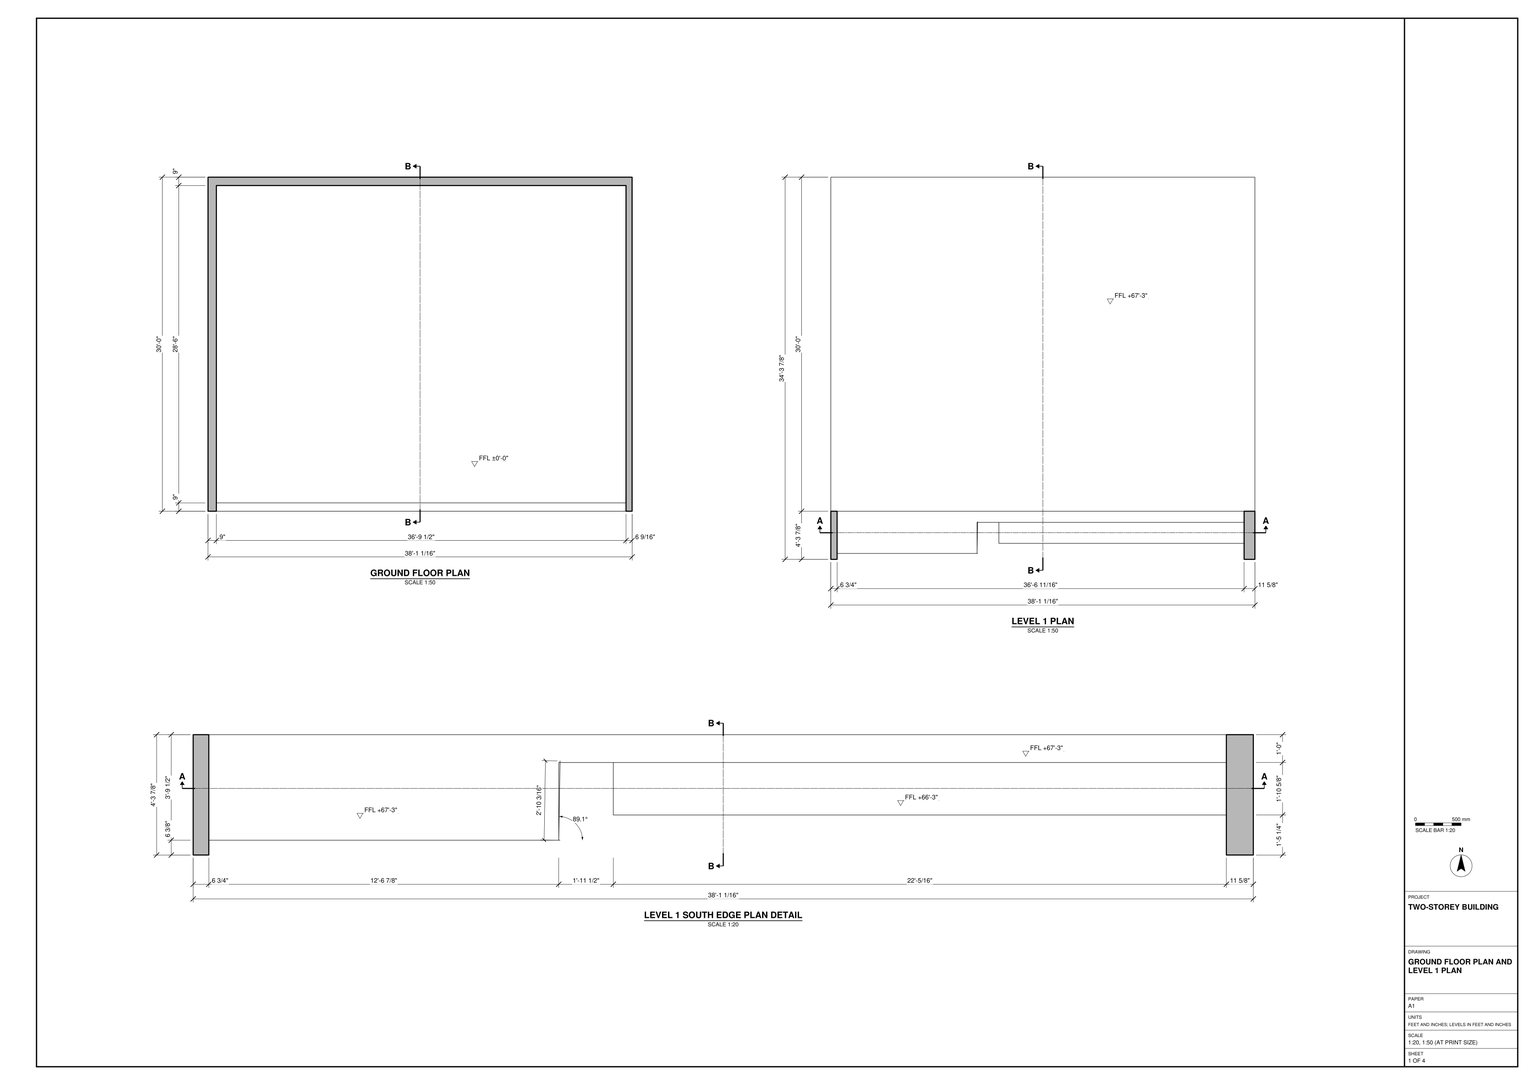
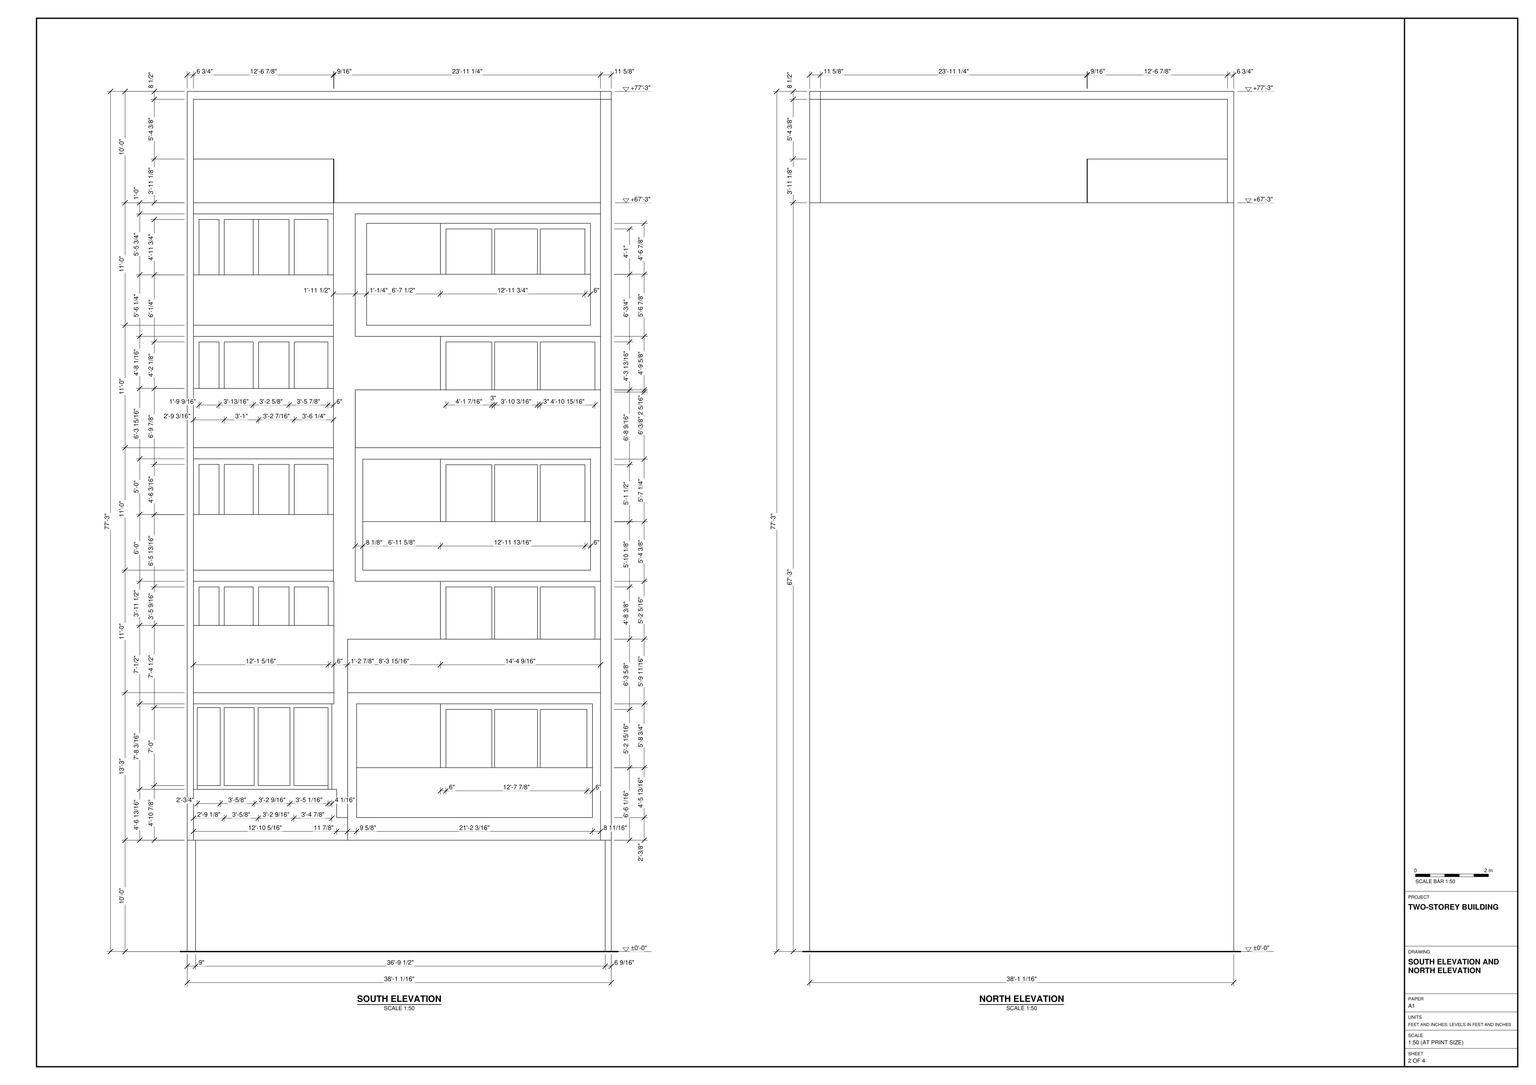
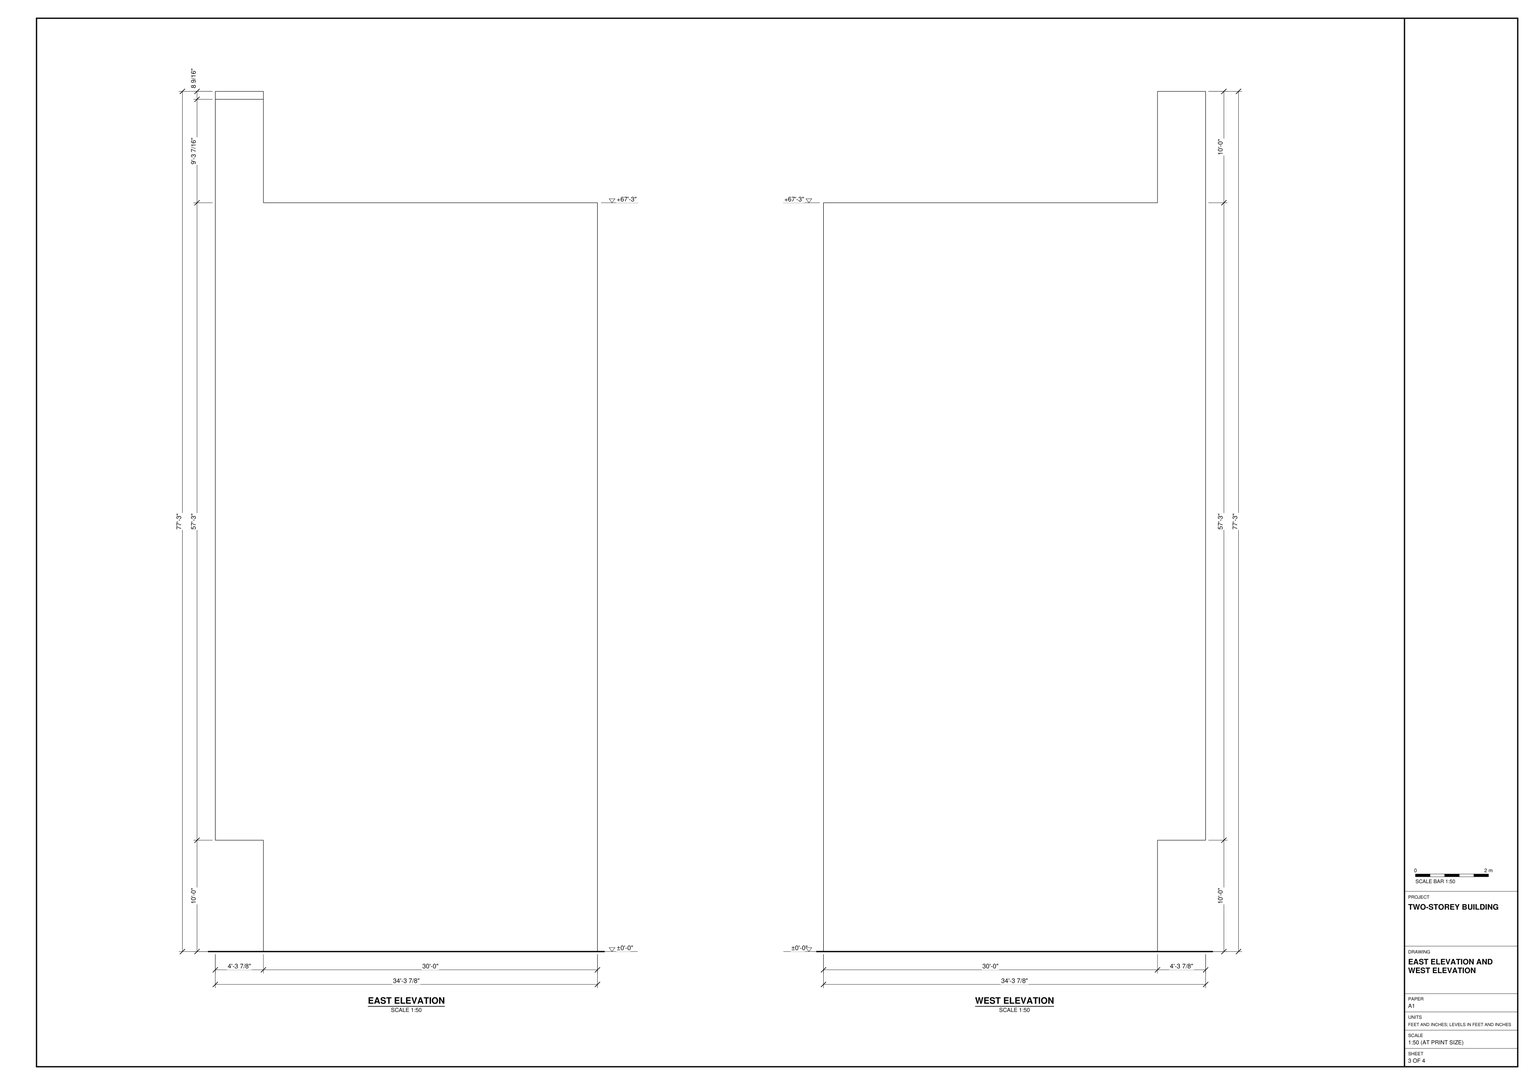
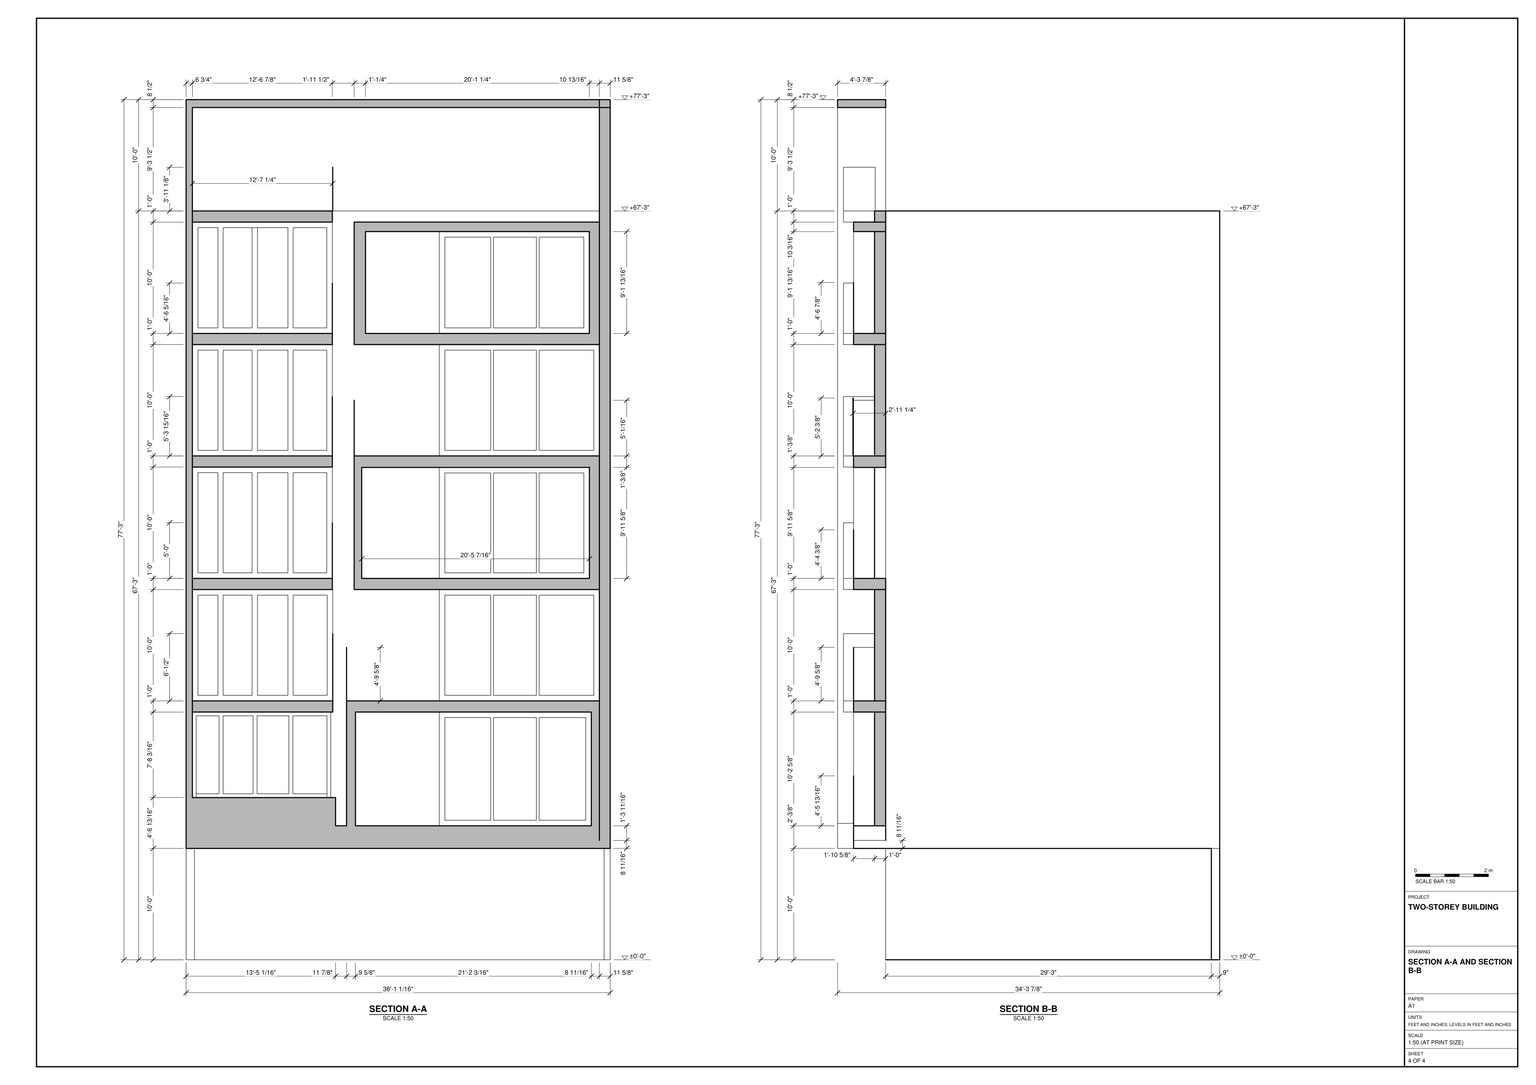
Build the two-storey building in SketchUp using task_files/diagram_01.pdf. Work in feet and inches. Set the overall width to 38'-1 1/16", depth to 34'-3 7/8" and height to 77'-3". Use ±0'-0" for the ground floor and +67'-3" for Level 1.

Start with the north wall and its two side returns, using the wall thicknesses in the ground floor plan. Keep the base open across the south between the returns. Above the base, project the south façade beyond the main wall line. Use the south elevation to lay out the five rows of window panels: the narrow left bay has closely spaced uprights, while the wider right bay has groups of panels set toward the right. Reproduce the solid bands between rows and the large rectangular surrounds on alternate rows. Keep the north, east and west wall faces plain as drawn.

Form the flat upper slab at Level 1. Use the enlarged south-edge plan for its changes in depth, and the elevations for the end returns and horizontal member that rise above it. Keep walls, slabs and façade assemblies in separate groups or components, and use components for repeated window units. Any decor or loose items shown may use suitable library components. Save one SketchUp model as output_files/two_storey_building_with_projecting_south_facade.skp.

# SketchUp Ruby script. Lengths in inches.
U = 1.inch
M = Sketchup.active_model
def pt(a) = Geom::Point3d.new(a.map { |v| v * U })
def face(e, loops, mat)
  f = e.add_face(loops[0].map { |a| pt(a) })
  loops[1..].each { |l| e.add_face(l.map { |a| pt(a) }).erase! }
  f.material = f.back_material = mat if mat
  f
end
# faces: each face lists its corners as indices into pts; further lists are holes
def faces(e, pts, list, mat = nil) = list.each { |f| face(e, (f[0].is_a?(Array) ? f : [f]).map { |l| l.map { |i| pts[i] } }, mat) }
# xy, xz, yz: faces in a plane at the given z, y or x. An outline is a flat list of corners, or four numbers for a rectangle; further outlines are holes
def ring(l) = l.size == 4 ? [[l[0], l[1]], [l[2], l[1]], [l[2], l[3]], [l[0], l[3]]] : l.each_slice(2).to_a
def flat(e, list, mat, &to3) = list.each { |f| face(e, (f[0].is_a?(Array) ? f : [f]).map { |l| ring(l).map { |u, v| to3.(u, v) } }, mat) }
def xy(e, z, list, mat = nil) = flat(e, list, mat) { |x, y| [x, y, z] }
def xz(e, y, list, mat = nil) = flat(e, list, mat) { |x, z| [x, y, z] }
def yz(e, x, list, mat = nil) = flat(e, list, mat) { |y, z| [x, y, z] }
def lines(e, pts, list) = list.each { |a, b| e.add_line(pt(pts[a]), pt(pts[b])) }
# prism: a flat outline (further loops are holes) pulled along v
def prism(e, loops, v, mat = nil)
  f = face(e, loops, mat); d = Geom::Vector3d.new(v.map { |x| x * U })
  f.pushpull(f.normal.samedirection?(d) ? d.length : -d.length)
end
def box(e, o, s, mat = nil) = prism(e, [[o, [o[0] + s[0], o[1], o[2]], [o[0] + s[0], o[1] + s[1], o[2]], [o[0], o[1] + s[1], o[2]]]], [0, 0, s[2]], mat)
def at(x, y, z, deg = 0) = Geom::Transformation.translation(pt([x, y, z])) * Geom::Transformation.rotation(ORIGIN, Z_AXIS, deg.degrees)
def axes(o, x, y, z) = Geom::Transformation.new([*x, 0, *y, 0, *z, 0, *pt(o).to_a, 1])
def part(name) = M.definitions.add(name)
# library, detail: a bought-in or finely detailed component or shape, given as its bounding box
def library(name, o, s) = part(name).tap { |d| box(d.entities, o, s) }
def detail(e, o, s) = box(e.add_group.entities, o, s)
def put(e, d, t, mat = nil) = e.add_instance(d, t).tap { |i| i.material = mat if mat }
def group(e, t, mat = nil) = e.add_group.tap { |g| g.transformation = t; g.material = mat if mat }.entities
root = M.entities
M.materials.add("[0035_Tan]").color = [178, 153, 119]
M.materials.add("[0137_Black]").color = [0, 0, 0]
M.materials.add("[Translucent Glass Gray]").color = [214, 214, 214]
M.materials["[Translucent Glass Gray]"].alpha = 0.5
M.materials.add("[Translucent Glass Gray]1").color = [181, 181, 181]
M.materials["[Translucent Glass Gray]1"].alpha = 0.5
M.materials.add("[Wood Lumber ButtJoined]").color = [150, 139, 102]
M.materials.add("[Wood Lumber ButtJoined]1").color = [164, 152, 112]
M.materials.add("[Wood OSB]").color = [183, 149, 93]
M.materials.add("[Wood OSB]1").color = [168, 136, 85]
xy(root,0,[[0,51.875,0,411.875,457.0625,411.875,457.0625,51.875,450.5,51.875,450.5,402.875,9,402.875,9,51.875],[9,51.875,450.5,60.875],[9,60.875,450.5,402.875]])
xy(root,120,[[0,0,6.74,51.875],[445.4375,0,457.0625,17.25],[6.74,17.25,457.0625,51.875],[9,51.875,450.5,402.875]])
xy(root,144.4,[[161.08,17.25,172.93,39.875],[182.56,17.25,436.74,17.25,436.74,45.875,272.88,45.875,272.88,39.875,182.56,39.875],[161.08,39.875,172.93,51.875],[182.56,39.875,272.88,51.875],[272.88,45.875,436.74,51.875]])
xy(root,150.4,[[278.88,45.875,328.32,51.875],[331.32,45.875,377.5,51.875],[380.5,45.875,430.74,51.875]],"[0137_Black]")
xy(root,174.8125,[[6.74,17.25,161.08,17.25,161.08,39.875,155.9,39.875,155.9,45.875,6.74,45.875],[155.9,39.875,161.08,51.875]])
xy(root,178.9,[[10.83,45.875,35.5625,51.875],[39.84,45.875,72.1875,51.875],[76.47,45.875,110.75,51.875],[115.03,45.875,151.82,51.875]],"[0137_Black]")
xy(root,261,[[278.88,45.875,328.32,51.875],[331.32,45.875,377.5,51.875],[380.5,45.875,430.74,51.875]],"[0137_Black]")
xy(root,262.92,[[10.83,45.875,35.5625,51.875],[39.84,45.875,72.1875,51.875],[76.47,45.875,110.75,51.875],[115.03,45.875,151.82,51.875]],"[0137_Black]")
xy(root,267,[[6.74,6.375,6.74,45.875,155.9,45.875,155.9,39.875,158.05,39.875,158.05,6.375],[182.56,39.875,272.88,51.875],[6.74,45.875,155.9,51.875],[272.88,45.875,436.74,51.875]])
xy(root,267,[[182.56,17.25,182.56,39.875,272.88,39.875,272.88,45.875,436.74,45.875,436.74,17.25]],"[Wood OSB]")
xy(root,279,[[6.74,6.375,158.05,45.875],[172.93,17.25,445.4375,17.25,445.4375,17.29],[172.93,17.25,445.4375,17.29,445.4375,45.875,272.88,45.875,272.88,39.875,172.93,39.875],[172.93,39.875,272.88,51.875],[6.74,45.875,158.05,51.875],
  [272.88,45.875,445.4375,51.875]])
xy(root,285,[[12.74,45.875,34.3,51.875],[39.93,45.875,71.12,51.875],[76.93,45.875,109.74,51.875],[115.37,45.875,152.05,51.875],[278.88,45.875,328.32,51.875],
  [331.32,45.875,377.5,51.875],[380.5,45.875,439.4375,51.875]],"[0137_Black]")
xy(root,393,[[12.74,45.875,34.3,51.875],[39.93,45.875,71.12,51.875],[76.93,45.875,109.74,51.875],[115.37,45.875,152.05,51.875],[278.88,45.875,328.32,51.875],
  [331.32,45.875,377.5,51.875],[380.5,45.875,439.4375,51.875]],"[0137_Black]")
xy(root,399,[[6.74,6.375,6.74,45.875,158.05,45.875,158.05,39.875,157.62,39.875,157.62,6.375],[181.13,39.875,189.25,51.875],[189.25,39.875,272.88,51.875],[6.74,45.875,158.05,51.875],[272.88,45.875,445.4375,51.875]])
xy(root,399,[[181.13,17.25,181.13,39.875,272.88,39.875,272.88,45.875,445.4375,45.875,445.4375,17.25]],"[Wood OSB]")
xy(root,411,[[6.74,6.375,157.62,45.875],[189.25,17.25,434.68,17.25,434.68,45.875,272.88,45.875,272.88,39.875,189.25,39.875],[189.25,39.875,272.88,51.875],[6.74,45.875,157.62,51.875],[272.88,45.875,434.68,51.875]])
xy(root,417,[[12.74,45.875,34.3,51.875],[39.93,45.875,71.12,51.875],[76.93,45.875,109.74,51.875],[115.37,45.875,151.62,51.875]])
xy(root,417,[[278.88,45.875,328.32,51.875],[331.32,45.875,377.5,51.875],[380.5,45.875,428.68,51.875]],"[0137_Black]")
xy(root,524.625,[[278.88,45.875,328.32,51.875],[331.32,45.875,377.5,51.875],[380.5,45.875,428.68,51.875]],"[0137_Black]")
xy(root,525,[[12.74,45.875,34.3,51.875],[39.93,45.875,71.12,51.875],[76.93,45.875,109.74,51.875],[115.37,45.875,151.62,51.875]],"[0137_Black]")
xy(root,530.625,[[189.25,39.875,272.88,51.875],[272.88,45.875,434.68,51.875]])
xy(root,530.625,[[189.25,17.25,189.25,39.875,272.88,39.875,272.88,45.875,434.68,45.875,434.68,17.25]],"[Wood OSB]")
xy(root,531,[[6.74,6.375,157.62,45.875],[6.74,45.875,157.62,51.875]])
xy(root,543,[[6.74,6.375,157.62,45.875],[181.13,17.25,181.2,39.875,181.13,39.875],[181.13,17.25,445.4375,17.25,445.4375,45.875,272.88,45.875,272.88,39.875,181.2,39.875],[181.13,39.875,189.25,51.875],[189.25,39.875,272.88,51.875],
  [6.74,45.875,157.62,51.875],[272.88,45.875,434.68,51.875],[434.68,45.875,445.4375,51.875]])
xy(root,549,[[12.74,45.875,34.3,51.875],[39.93,45.875,71.12,51.875],[76.93,45.875,109.74,51.875],[115.37,45.875,151.62,51.875],[278.88,45.875,328.32,51.875],
  [331.32,45.875,377.5,51.875],[380.5,45.875,434.68,51.875],[434.68,45.875,439.4375,51.875]],"[0137_Black]")
xy(root,657,[[12.74,45.875,34.3,51.875],[39.93,45.875,71.12,51.875],[76.93,45.875,109.74,51.875],[115.37,45.875,151.62,51.875],[278.88,45.875,328.32,51.875],
  [331.32,45.875,377.5,51.875],[380.5,45.875,439.4375,51.875]],"[0137_Black]")
xy(root,663,[[6.74,6.375,157.62,45.875],[181.13,39.875,272.88,51.875],[6.74,45.875,157.62,51.875],[272.88,45.875,445.4375,51.875]])
xy(root,663,[[181.13,17.25,181.13,39.875,272.88,39.875,272.88,45.875,445.4375,45.875,445.4375,17.25]],"[Wood OSB]")
xy(root,675,[[6.74,6.375,157.62,45.875],[193.35,17.25,434.625,17.25,434.625,45.875,272.88,45.875,272.88,39.875,193.35,39.875],[193.35,39.875,272.88,51.875],[6.74,45.875,157.62,51.875],[272.88,45.875,434.625,51.875]])
xy(root,681,[[12.74,45.875,34.3,51.875],[39.93,45.875,71.12,51.875],[76.93,45.875,109.74,51.875],[115.37,45.875,151.62,51.875],[278.88,45.875,328.32,51.875],
  [331.32,45.875,377.5,51.875],[380.5,45.875,428.625,51.875]],"[0137_Black]")
xy(root,778.79,[[278.88,45.875,328.32,51.875],[331.32,45.875,377.5,51.875],[380.5,45.875,428.625,51.875]],"[0137_Black]")
xy(root,784.79,[[193.35,39.875,272.88,51.875],[272.88,45.875,434.625,51.875]])
xy(root,784.79,[[193.35,17.25,193.35,39.875,272.88,39.875,272.88,45.875,434.625,45.875,434.625,17.25]],"[Wood OSB]")
xy(root,789,[[71.12,45.875,76.93,51.875]])
xy(root,789,[[12.74,45.875,34.3,51.875],[39.93,45.875,71.12,51.875],[76.93,45.875,109.74,51.875],[115.37,45.875,151.62,51.875]],"[0137_Black]")
xy(root,795,[[6.74,6.375,157.62,45.875],[181.13,39.875,445.4375,51.875],[6.74,45.875,157.62,51.875]])
xy(root,795,[[181.13,17.25,445.4375,39.875]],"[Wood OSB]1")
xy(root,807,[[6.74,6.375,157.62,6.375,157.62,39.875,445.4375,39.875,445.4375,51.875,6.74,51.875],[157.62,6.375,158.17,39.875,157.62,39.875]])
xy(root,807,[[0,51.875,457.0625,411.875]],"[0035_Tan]")
xy(root,918.48,[[6.74,0,457.0625,51.875]],"[0035_Tan]")
xy(root,927,[[0,0,445.4375,51.875],[445.4375,0,457.0625,51.875]],"[0035_Tan]")
xz(root,0,[[0,120,6.74,120,6.74,918.48,445.4375,918.48,445.4375,927,0,927],[445.4375,120,457.0625,918.48],[445.4375,918.48,457.0625,927]],"[0035_Tan]")
xz(root,6.375,[[6.74,267,158.05,279],[6.74,399,157.62,411],[6.74,531,157.62,543],[6.74,663,157.62,675],[6.74,795,157.62,807],
  [157.62,807,158.18,854.125]])
xz(root,6.375,[[6.74,279,158.05,351.5],[6.74,411,157.62,471],[6.74,543,157.62,606.91],[6.74,675,157.62,729.27],[6.74,807,157.62,854.125]],"[Translucent Glass Gray]1")
xz(root,17.25,[[6.74,120,172.93,120,172.93,144.4,161.08,144.4,161.08,174.8125,6.74,174.8125]])
xz(root,17.25,[[182.56,144.4,436.74,198.22],[189.25,411,434.68,463.375],[193.35,675,434.625,729.9]],"[Translucent Glass Gray]")
xz(root,17.25,[[[172.93,120,445.4375,279],[182.56,144.4,436.74,267]],[[181.13,399,445.4375,543],[189.25,411,434.68,530.625]],[[181.13,663,445.4375,795],[193.35,675,434.625,784.79]]],"[Wood OSB]")
xz(root,39.875,[[161.08,144.4,172.93,144.4,172.93,279,272.88,279,272.88,399,181.13,399,181.13,543,272.88,543,272.88,663,181.13,663,181.13,795,445.4375,795,445.4375,807,157.62,807,157.62,399,158.05,399,158.05,267,155.9,267,155.9,174.8125,161.08,174.8125],[189.25,411,272.88,530.625]],"[Wood Lumber ButtJoined]")
xz(root,39.875,[[182.56,144.4,272.88,267],[193.35,675,272.88,784.79]],"[Wood Lumber ButtJoined]1")
xz(root,45.875,[[[272.88,144.4,436.74,267],[380.5,150.4,430.74,261],[278.88,150.4,328.32,261],[331.32,150.4,377.5,261]],[[6.74,174.8125,10.83,174.8125,10.83,262.92,35.5625,262.92,35.5625,178.9,10.83,178.9,10.83,174.8125,151.82,174.8125,151.82,178.9,115.03,178.9,115.03,262.92,151.82,262.92,151.82,174.8125,155.9,174.8125,155.9,267,6.74,267],[76.47,178.9,110.75,262.92],[39.84,178.9,72.1875,262.92]],[[6.74,279,158.05,399],[115.37,285,152.05,393],[76.93,285,109.74,393],[39.93,285,71.12,393],[12.74,285,34.3,393]],[[272.88,279,445.4375,399],[380.5,285,439.4375,393],[278.88,285,328.32,393],[331.32,285,377.5,393]],[[6.74,411,157.62,531],[115.37,417,151.62,525],[76.93,417,109.74,525],[39.93,417,71.12,525],[12.74,417,34.3,525]],
  [[272.88,411,434.68,530.625],[278.88,417,328.32,524.625],[380.5,417,428.68,524.625],[331.32,417,377.5,524.625]],[[6.74,543,157.62,663],[115.37,549,151.62,657],[76.93,549,109.74,657],[39.93,549,71.12,657],[12.74,549,34.3,657]],[[272.88,543,445.4375,663],[380.5,549,439.4375,657],[278.88,549,328.32,657],[331.32,549,377.5,657]],[[6.74,675,157.62,795],[39.93,681,39.93,789,109.74,789,109.74,681,76.93,681,76.93,789,71.12,789,71.12,681],[115.37,681,151.62,789],[12.74,681,34.3,789]],[[272.88,675,434.625,784.79],[278.88,681,328.32,778.79],[380.5,681,428.625,778.79],[331.32,681,377.5,778.79]]],"[0137_Black]")
xz(root,51.875,[[0,0,9,120],[450.5,0,457.0625,120],[161.08,128.6875,161.08,144.4,436.74,144.4,436.74,267,445.4375,267,445.4375,128.6875],[161.08,144.4,161.08,174.8125,155.9,174.8125,155.9,267,167.02,267,167.02,279,158.05,279,158.05,399,169.9,399,169.9,411,157.62,411,157.62,531,169.9,531,169.9,543,157.62,543,157.62,663,169.9,663,169.9,675,157.62,675,157.62,795,169.9,795,169.9,807,445.4375,807,445.4375,795,181.13,795,181.13,663,272.88,663,272.88,543,181.13,543,181.13,399,272.88,399,272.88,279,172.93,279,172.93,144.4],[172.93,144.4,182.56,263.96],
  [182.56,144.4,272.88,267],[[272.88,144.4,436.74,267],[380.5,150.4,430.74,261],[278.88,150.4,328.32,261],[331.32,150.4,377.5,261]],[172.93,263.96,182.56,267],[6.74,267,167.02,279],[172.93,267,445.4375,279],
  [[272.88,279,445.4375,399],[380.5,285,439.4375,393],[278.88,285,328.32,393],[331.32,285,377.5,393]],[6.74,399,169.9,411],[181.13,399,189.25,411],[189.25,399,189.25,411,434.68,411,434.68,531,445.4375,531,445.4375,399],[181.13,411,189.25,531],
  [[272.88,411,434.68,530.625],[278.88,417,328.32,524.625],[380.5,417,428.68,524.625],[331.32,417,377.5,524.625]],[189.25,530.625,434.68,531],[6.74,531,169.9,543],[181.13,531,189.25,543],[189.25,531,434.68,543],
  [434.68,531,445.4375,543],[[272.88,543,445.4375,663],[380.5,549,439.4375,657],[278.88,549,328.32,657],[331.32,549,377.5,657]],[6.74,663,169.9,675],[[181.13,663,445.4375,795],[193.35,675,434.625,784.79]],[193.35,675,272.88,784.79],
  [6.74,795,169.9,807]])
xz(root,51.875,[[0,807,0,927,445.4375,927,445.4375,918.48,6.74,918.48,6.74,807],[445.4375,807,457.0625,918.48],[445.4375,918.48,457.0625,927]],"[0035_Tan]")
xz(root,51.875,[[278.88,150.4,328.32,261],[331.32,150.4,377.5,261],[380.5,150.4,430.74,261],[10.83,178.9,35.5625,262.92],[39.84,178.9,72.1875,262.92],
  [76.47,178.9,110.75,262.92],[115.03,178.9,151.82,262.92],[12.74,285,34.3,393],[39.93,285,71.12,393],[76.93,285,109.74,393],
  [115.37,285,152.05,393],[278.88,285,328.32,393],[331.32,285,377.5,393],[380.5,285,439.4375,393],[12.74,417,34.3,525],
  [39.93,417,71.12,525],[76.93,417,109.74,525],[115.37,417,151.62,525],[278.88,417,328.32,524.625],[331.32,417,377.5,524.625],
  [380.5,417,428.68,524.625],[12.74,549,34.3,657],[39.93,549,71.12,657],[76.93,549,109.74,657],[115.37,549,151.62,657],
  [278.88,549,328.32,657],[331.32,549,377.5,657],[380.5,549,439.4375,657],[12.74,681,34.3,789],[39.93,681,71.12,789],
  [76.93,681,109.74,789],[115.37,681,151.62,789],[278.88,681,328.32,778.79],[331.32,681,377.5,778.79],[380.5,681,428.625,778.79]],"[Translucent Glass Gray]1")
xz(root,402.875,[[9,0,450.5,120]])
xz(root,411.875,[[0,0,457.0625,807]],"[0035_Tan]")
yz(root,0,[[51.875,0,51.875,120,0,120,0,927,51.875,927,51.875,807,411.875,807,411.875,0]],"[0035_Tan]")
yz(root,6.74,[[6.375,267,51.875,279],[6.375,399,51.875,411],[6.375,531,51.875,543],[6.375,663,51.875,675],[6.375,795,51.875,807]])
yz(root,6.74,[[0,120,17.25,147],[0,147,17.25,147,17.25,174.8125,45.875,174.8125,45.875,267,6.375,267,6.375,279,45.875,279,45.875,399,6.375,399,6.375,411,45.875,411,45.875,531,6.375,531,6.375,543,45.875,543,45.875,663,6.375,663,6.375,675,45.875,675,45.875,795,6.375,795,6.375,807,51.875,807,51.875,918.48,0,918.48]],"[0035_Tan]")
yz(root,9,[[51.875,0,402.875,120]])
yz(root,10.83,[[45.875,174.8125,48.875,178.9],[48.875,174.8125,48.875,178.9,51.875,178.9]])
yz(root,10.83,[[45.875,178.9,51.875,262.92]],"[0137_Black]")
yz(root,12.74,[[45.875,285,51.875,393],[45.875,417,51.875,525],[45.875,549,51.875,657],[45.875,681,51.875,789]],"[0137_Black]")
yz(root,34.3,[[45.875,285,51.875,393],[45.875,417,51.875,525],[45.875,549,51.875,657],[45.875,681,51.875,789]],"[0137_Black]")
yz(root,35.5625,[[45.875,178.9,51.875,262.92]],"[0137_Black]")
yz(root,39.84,[[45.875,178.9,51.875,262.92]],"[0137_Black]")
yz(root,39.93,[[45.875,285,51.875,393],[45.875,417,51.875,525],[45.875,549,51.875,657],[45.875,681,51.875,789]],"[0137_Black]")
yz(root,71.12,[[45.875,285,51.875,393],[45.875,417,51.875,525],[45.875,549,51.875,657],[45.875,681,51.875,789]],"[0137_Black]")
yz(root,72.1875,[[45.875,178.9,51.875,262.92]],"[0137_Black]")
yz(root,76.47,[[45.875,178.9,51.875,262.92]],"[0137_Black]")
yz(root,76.93,[[45.875,285,51.875,393],[45.875,417,51.875,525],[45.875,549,51.875,657],[45.875,681,51.875,789]],"[0137_Black]")
yz(root,109.74,[[45.875,285,51.875,393],[45.875,417,51.875,525],[45.875,549,51.875,657],[45.875,681,51.875,789]],"[0137_Black]")
yz(root,110.75,[[45.875,178.9,51.875,262.92]],"[0137_Black]")
yz(root,115.03,[[45.875,178.9,51.875,262.92]],"[0137_Black]")
yz(root,115.37,[[45.875,285,51.875,393],[45.875,417,51.875,525],[45.875,549,51.875,657],[45.875,681,51.875,789]],"[0137_Black]")
yz(root,151.62,[[45.875,417,51.875,525],[45.875,549,51.875,657],[45.875,681,51.875,789]],"[0137_Black]")
yz(root,151.82,[[45.875,174.8125,48.875,178.9],[48.875,174.8125,51.875,178.9,48.875,178.9]])
yz(root,151.82,[[45.875,178.9,51.875,262.92]],"[0137_Black]")
yz(root,152.05,[[45.875,285,51.875,393]],"[0137_Black]")
yz(root,155.9,[[45.875,174.8125,51.875,267]])
yz(root,155.9,[[39.875,174.8125,45.875,267]],"[Wood Lumber ButtJoined]1")
yz(root,157.62,[[6.375,399,39.875,411],[39.875,411,45.875,471],[45.875,411,51.875,531],[6.375,531,39.875,543],[39.875,543,45.875,606.91],
  [45.875,543,51.875,663],[6.375,663,39.875,675],[39.875,675,45.875,729.27],[45.875,675,51.875,795],[6.375,795,39.875,807]])
yz(root,157.62,[[6.375,411,39.875,471],[6.375,543,39.875,606.91],[6.375,675,39.875,729.27]],"[Translucent Glass Gray]1")
yz(root,157.62,[[39.875,471,45.875,531],[39.875,606.91,45.875,663],[39.875,729.27,45.875,795]],"[Wood Lumber ButtJoined]")
yz(root,158.05,[[6.375,267,39.875,279],[39.875,279,45.875,351.5],[45.875,279,51.875,399]])
yz(root,158.05,[[6.375,279,39.875,351.5]],"[Translucent Glass Gray]1")
yz(root,158.05,[[39.875,351.5,45.875,399]],"[Wood Lumber ButtJoined]")
yz(root,161.08,[[17.25,144.4,39.875,174.8125],[39.875,144.4,51.875,174.8125]])
yz(root,172.93,[[39.875,144.4,51.875,263.96],[39.875,263.96,51.875,267],[39.875,267,51.875,279]])
yz(root,172.93,[[17.25,279,39.875,336.66]],"[Translucent Glass Gray]")
yz(root,172.93,[[17.25,144.4,39.875,279]],"[Wood OSB]")
yz(root,181.13,[[39.875,399,51.875,411],[39.875,411,51.875,531],[39.875,531,51.875,543],[39.875,663,51.875,795]])
yz(root,181.13,[[17.25,399,39.875,543],[17.25,663,39.875,795]],"[Wood OSB]")
yz(root,182.56,[[39.875,144.4,51.875,263.96],[39.875,263.96,51.875,267]])
yz(root,182.56,[[17.25,144.4,39.875,267]],"[Wood OSB]")
yz(root,189.25,[[39.875,411,51.875,530.625]])
yz(root,189.25,[[17.25,411,39.875,530.625]],"[Wood OSB]")
yz(root,193.35,[[39.875,675,51.875,784.79]])
yz(root,193.35,[[17.25,675,39.875,784.79]],"[Wood OSB]")
yz(root,272.88,[[45.875,144.4,51.875,267],[45.875,279,51.875,399],[45.875,411,51.875,530.625],[45.875,543,51.875,663],[45.875,675,51.875,784.79]])
yz(root,272.88,[[39.875,279,45.875,399],[39.875,411,45.875,530.625],[39.875,543,45.875,663]],"[Wood Lumber ButtJoined]")
yz(root,272.88,[[39.875,144.4,45.875,267],[39.875,675,45.875,784.79]],"[Wood Lumber ButtJoined]1")
yz(root,278.88,[[45.875,150.4,51.875,261],[45.875,285,51.875,393],[45.875,417,51.875,524.625],[45.875,549,51.875,657],[45.875,681,51.875,778.79]],"[0137_Black]")
yz(root,328.32,[[45.875,150.4,51.875,261],[45.875,285,51.875,393],[45.875,417,51.875,524.625],[45.875,549,51.875,657],[45.875,681,51.875,778.79]],"[0137_Black]")
yz(root,331.32,[[45.875,150.4,51.875,261],[45.875,285,51.875,393],[45.875,417,51.875,524.625],[45.875,549,51.875,657],[45.875,681,51.875,778.79]],"[0137_Black]")
yz(root,377.5,[[45.875,150.4,51.875,261],[45.875,285,51.875,393],[45.875,417,51.875,524.625],[45.875,549,51.875,657],[45.875,681,51.875,778.79]],"[0137_Black]")
yz(root,380.5,[[45.875,150.4,51.875,261],[45.875,285,51.875,393],[45.875,417,51.875,524.625],[45.875,549,51.875,657],[45.875,681,51.875,778.79]],"[0137_Black]")
yz(root,428.625,[[45.875,681,51.875,778.79]],"[0137_Black]")
yz(root,428.68,[[45.875,417,51.875,524.625]],"[0137_Black]")
yz(root,430.74,[[45.875,150.4,51.875,261]],"[0137_Black]")
yz(root,434.625,[[45.875,675,51.875,784.79]])
yz(root,434.625,[[17.25,675,45.875,784.79]],"[Wood OSB]")
yz(root,434.68,[[45.875,411,51.875,530.625],[17.25,530.625,51.875,531]])
yz(root,434.68,[[17.25,411,45.875,530.625]],"[Wood OSB]")
yz(root,436.74,[[45.875,144.4,51.875,267]])
yz(root,436.74,[[17.25,144.4,45.875,267]],"[Wood OSB]")
yz(root,439.4375,[[45.875,285,51.875,393],[45.875,549,51.875,657]],"[0137_Black]")
yz(root,445.4375,[[17.25,128.6875,51.875,267],[17.25,267,51.875,279],[45.875,279,51.875,399],[17.25,399,51.875,531],[17.25,531,51.875,543],
  [45.875,543,51.875,663],[17.25,663,51.875,795],[39.875,795,51.875,807]])
yz(root,445.4375,[[0,120,0,927,51.875,927,51.875,807,39.875,807,39.875,795,17.25,795,17.25,663,45.875,663,45.875,543,17.25,543,17.25,399,45.875,399,45.875,279,17.25,279,17.25,120]],"[0035_Tan]")
yz(root,450.5,[[51.875,0,402.875,120]])
yz(root,457.0625,[[51.875,0,411.875,0,411.875,807,51.875,807,51.875,918.48,0,918.48,0,120,51.875,120],[0,918.48,51.875,927]],"[0035_Tan]")
p = [[445.4375,17.29,279],[172.93,17.25,279],[172.93,17.25,336.66],[445.4375,17.29,336.66],[181.13,17.25,543],[445.4375,13.84,543],
  [445.4375,13.84,605.37],[181.13,17.25,605.37],[181.13,17.25,603.03],[181.2,39.875,543],[181.2,39.875,603.03],[158.17,39.875,807],
  [157.62,6.375,807],[157.62,6.375,854.125],[158.18,40.5625,854.125],[158.18,40.5625,807],[9,402.875,120],[0,402.875,120],
  [9,60.875,120],[0,60.875,120],[9,411.875,120],[167.02,51.875,267],[167.02,39.875,267],[167.02,51.875,279],
  [167.02,39.875,279],[169.9,51.875,399],[169.9,39.875,399],[169.9,51.875,411],[169.9,39.875,411],[169.9,51.875,531],
  [169.9,39.875,531],[169.9,51.875,543],[169.9,39.875,543],[169.9,51.875,663],[169.9,39.875,663],[169.9,51.875,675],
  [169.9,39.875,675],[169.9,51.875,795],[169.9,39.875,795],[161.08,51.875,128.6875],[161.08,17.25,128.6875],[189.25,51.875,531],
  [189.25,17.25,531]]
faces(root,p,[[0,1,2,3],[4,5,6,7,8],[9,4,8,10]],"[Translucent Glass Gray]")
faces(root,p,[[11,12,13,14,15]],"[Translucent Glass Gray]1")
lines(root,p,[[16,17],[18,19],[16,20],[21,22],[23,24],[25,26],[27,28],[29,30],[31,32],[33,34],[35,36],[37,38],
  [39,40],[41,42]])
